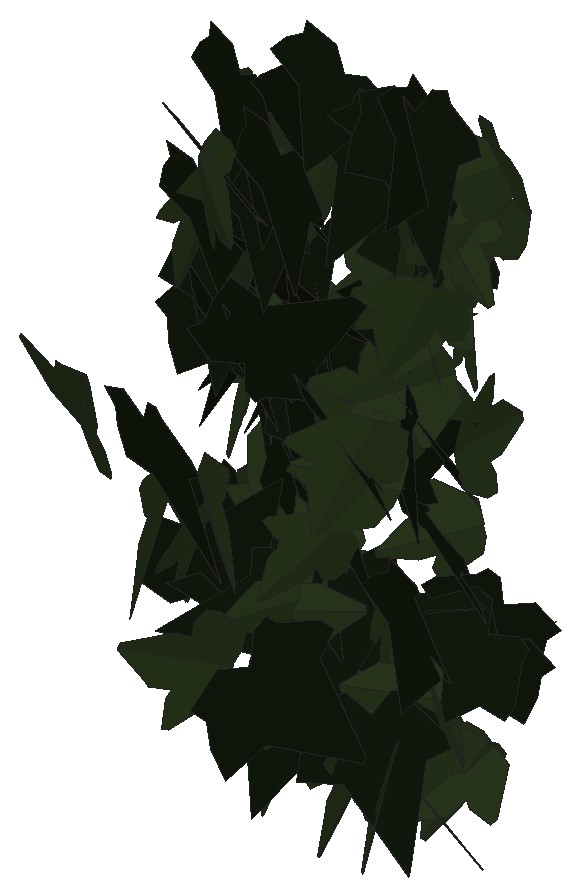
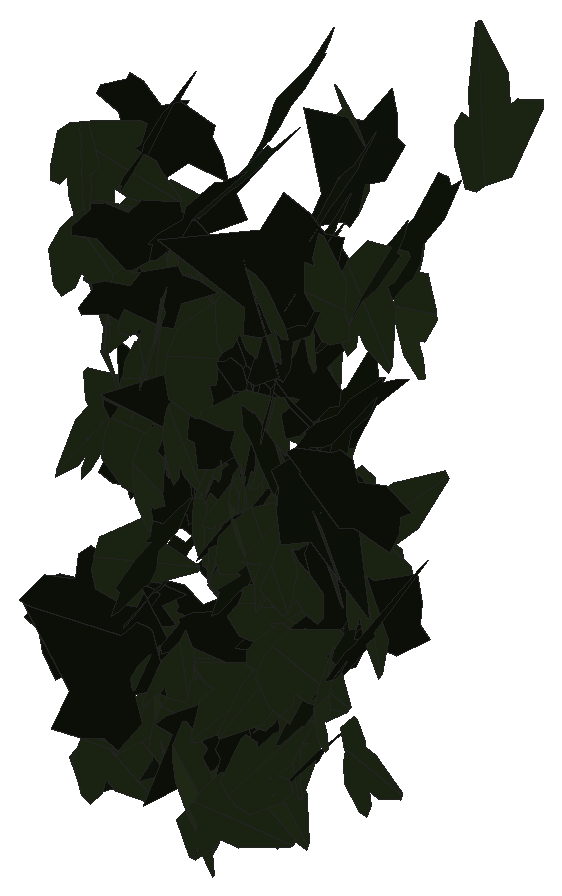
# SketchUp Ruby script. Lengths in inches.
U = 1.inch
M = Sketchup.active_model
def pt(a) = Geom::Point3d.new(a.map { |v| v * U })
def face(e, loops, mat)
  f = e.add_face(loops[0].map { |a| pt(a) })
  loops[1..].each { |l| e.add_face(l.map { |a| pt(a) }).erase! }
  f.material = f.back_material = mat if mat
  f
end
# faces: each face lists its corners as indices into pts; further lists are holes
def faces(e, pts, list, mat = nil) = list.each { |f| face(e, (f[0].is_a?(Array) ? f : [f]).map { |l| l.map { |i| pts[i] } }, mat) }
# xy, xz, yz: faces in a plane at the given z, y or x. An outline is a flat list of corners, or four numbers for a rectangle; further outlines are holes
def ring(l) = l.size == 4 ? [[l[0], l[1]], [l[2], l[1]], [l[2], l[3]], [l[0], l[3]]] : l.each_slice(2).to_a
def flat(e, list, mat, &to3) = list.each { |f| face(e, (f[0].is_a?(Array) ? f : [f]).map { |l| ring(l).map { |u, v| to3.(u, v) } }, mat) }
def xy(e, z, list, mat = nil) = flat(e, list, mat) { |x, y| [x, y, z] }
def xz(e, y, list, mat = nil) = flat(e, list, mat) { |x, z| [x, y, z] }
def yz(e, x, list, mat = nil) = flat(e, list, mat) { |y, z| [x, y, z] }
def lines(e, pts, list) = list.each { |a, b| e.add_line(pt(pts[a]), pt(pts[b])) }
# prism: a flat outline (further loops are holes) pulled along v
def prism(e, loops, v, mat = nil)
  f = face(e, loops, mat); d = Geom::Vector3d.new(v.map { |x| x * U })
  f.pushpull(f.normal.samedirection?(d) ? d.length : -d.length)
end
def box(e, o, s, mat = nil) = prism(e, [[o, [o[0] + s[0], o[1], o[2]], [o[0] + s[0], o[1] + s[1], o[2]], [o[0], o[1] + s[1], o[2]]]], [0, 0, s[2]], mat)
def at(x, y, z, deg = 0) = Geom::Transformation.translation(pt([x, y, z])) * Geom::Transformation.rotation(ORIGIN, Z_AXIS, deg.degrees)
def axes(o, x, y, z) = Geom::Transformation.new([*x, 0, *y, 0, *z, 0, *pt(o).to_a, 1])
def part(name) = M.definitions.add(name)
# library, detail: a bought-in or finely detailed component or shape, given as its bounding box
def library(name, o, s) = part(name).tap { |d| box(d.entities, o, s) }
def detail(e, o, s) = box(e.add_group.entities, o, s)
def put(e, d, t, mat = nil) = e.add_instance(d, t).tap { |i| i.material = mat if mat }
def group(e, t, mat = nil) = e.add_group.tap { |g| g.transformation = t; g.material = mat if mat }.entities
root = M.entities
M.materials.add("efeu1").color = [18, 25, 13]
M.materials.add("efeu2").color = [43, 57, 29]
c1 = part("ivyleaf_10")
p = [[0,0.5,-0.03],[-0.0625,2.02,-0.43],[-0.19,2.01,-0.46],[-0.54,1.05,-0.29],[-0.52,0.625,-0.18],[-0.83,0.76,-0.28],
  [-1.16,0.64,-0.33],[-1.15,0.33,-0.24],[-0.77,-0.39,0.02],[-0.3,-0.51,0.16],[0.04,-0.48,0.23],[-0.02,2.01,-0.4375],
  [-0.06,2.01,-0.43],[0.04,-0.49,0.23],[0.67,-0.49,0.14],[1.38,0.36,-0.2],[1.375,0.51,-0.24],[0.81,0.65,-0.19],
  [0.62,0.59,-0.15],[0.6,1.09,-0.28],[0.5,1.23,-0.31]]
faces(c1.entities,p,[[0,1,2,3,4,5,6,7,8,9,10],[11,12,0,13,14,15,16,17,18,19,20]],"efeu2")
c2 = part("ivyleaf_9")
p = [[1.54,2.16,1.25],[1.36,2.04,1.19],[-0.21,0.99,0.68],[-0.71,1.11,0.82],[-0.85,0.86,0.67],[-0.8,0.17,0.21],
  [-0.9,-0.01,0.1],[-0.67,-0.16,-0.02],[-0.08,-0.08,-0.05],[-0.03,-0.6,-0.4],[0.65,-0.88,-0.66],[0.83,-0.6,-0.49],
  [1.29,-0.42,-0.43],[1.8125,-0.07,-0.26],[1.21,0.44,0.15]]
faces(c2.entities,p,[[0,1,2,3,4,5,6,7,8,9,10,11,12,13,14]],"efeu1")
put(root,c1,axes([521.53,128.375,181.19],[-0.85624,0.15048,0.62072],[0.56209,-0.31547,0.85184],[0.30331,1.00942,0.17368]))
put(root,c1,axes([521.82,130.08,178.96],[0.25692,-0.3956,0.84112],[0.51271,-0.66758,-0.47059],[0.77531,0.57256,0.03248]))
put(root,c2,axes([521.51,130.16,180.27],[0.564,-0.75753,0.18315],[0.11068,-0.14594,-0.94443],[0.77146,0.57475,0.0016]))
put(root,c1,axes([521.68,131.56,175.45],[-0.18984,-0.2558,-0.80001],[-0.49065,-0.63191,0.31848],[-0.68169,0.52606,-0.00644]))
put(root,c2,axes([522.62,131.46,175.6875],[0.12859,-0.32835,-0.91099],[-0.21634,0.88602,-0.34989],[0.94388,0.24781,0.04391]))
put(root,c1,axes([521.26,132.04,178.09],[-0.47981,0.69752,0.08512],[-0.04953,0.06925,-0.84661],[-0.70095,-0.48236,0.00156]))
put(root,c1,axes([520.76,132.68,183.39],[-0.20173,0.08556,-0.81779],[0.49347,-0.66094,-0.19087],[-0.65771,-0.52214,0.10761]))
put(root,c1,axes([523.77,132.73,179.65],[-0.39116,-0.67084,0.38941],[-0.11622,-0.38051,-0.77226],[0.76692,-0.39982,0.08158]))
put(root,c2,axes([521.96,132.93,183.94],[0.23926,-0.74582,0.36603],[0.08109,-0.35812,-0.78272],[0.82683,0.25094,-0.02915]))
put(root,c2,axes([522.88,133.11,179.41],[0.29561,-0.55547,0.55692],[0.36081,-0.43291,-0.6233],[0.69894,0.45841,0.08621]))
put(root,c2,axes([520.23,133.24,183.27],[0.22099,-0.49408,0.66016],[0.45648,-0.49587,-0.52393],[0.6867,0.48863,0.13583]))
put(root,c1,axes([523.62,133.49,173.44],[0.53015,-0.61555,0.24235],[0.15312,-0.18795,-0.81236],[0.64357,0.55179,-0.00635]))
put(root,c2,axes([521.26,133.03,180.08],[-0.05232,-0.01524,0.84946],[0.84681,-0.06992,0.0509],[0.06887,0.8482,0.01946]))
put(root,c2,axes([523.47,133.32,174.27],[-0.36679,-0.49197,-0.58723],[0.35546,0.46744,-0.61364],[0.67862,-0.51076,0.00403]))
put(root,c1,axes([522.92,133.78,173.35],[0.22016,-0.65504,0.51825],[0.17005,-0.48957,-0.69103],[0.81776,0.27815,0.00417]))
put(root,c1,axes([522.21,133.6875,176.93],[-0.25975,-0.43298,0.49778],[-0.24936,-0.43086,-0.50489],[0.6108,-0.36003,0.00557]))
put(root,c1,axes([523.02,133.96,178.05],[0.04142,0.41072,0.69902],[-0.12808,-0.68783,0.41173],[0.80057,-0.1313,0.0297]))
put(root,c1,axes([521.35,134.22,175.35],[0.00535,0.07548,0.79166],[-0.02054,-0.7914,0.07559],[0.79498,-0.02096,-0.00338]))
put(root,c2,axes([521.42,134.17,175.21],[-0.12864,-0.31702,-0.71842],[-0.31596,-0.64557,0.34145],[-0.71889,0.34046,-0.02151]))
put(root,c1,axes([519.73,133.77,176.43],[0.13839,-0.83853,-0.06256],[-0.01138,0.06153,-0.84988],[0.84079,0.13885,-0.0012]))
put(root,c2,axes([519.41,134.3,181.83],[0.19789,-0.72797,0.42536],[0.17769,-0.3911,-0.752],[0.8242,0.2591,0.06]))
put(root,c2,axes([519.8,133.7,175.1875],[-0.37067,-0.1078,0.73364],[0.73908,-0.12015,0.35576],[0.06007,0.81313,0.14983]))
put(root,c1,axes([523.99,133.98,181.66],[-0.52596,-0.47765,0.32754],[-0.24717,-0.21501,-0.71046],[0.52378,-0.58111,-0.00636]))
put(root,c1,axes([521.04,133.76,173.81],[0.07599,-0.79622,-0.29415],[-0.03191,0.29244,-0.79983],[0.84822,0.08233,-0.00374]))
put(root,c1,axes([519.47,134.27,182.06],[0.10925,-0.81636,0.27169],[0.07847,-0.26328,-0.82263],[0.8568,0.1282,0.0407]))
put(root,c1,axes([520.4,134.18,181.11],[0.20781,-0.69335,0.09716],[0.03159,-0.09196,-0.72381],[0.69941,0.21017,0.00383]))
put(root,c2,axes([520.39,134.51,182.125],[0.08087,-0.70528,0.31233],[0.07837,-0.3049,-0.7088],[0.76735,0.10547,0.03947]))
put(root,c1,axes([520.95,134.02,175.13],[0.15316,-0.01523,-0.79976],[0.79856,-0.04419,0.15377],[-0.04627,-0.81309,0.00662]))
put(root,c1,axes([522.4,134.49,178.82],[-0.13144,0.57468,0.54752],[0.08748,-0.5411,0.58895],[0.78891,0.15575,0.02591]))
put(root,c1,axes([523.69,134.3,174.36],[-0.09119,0.13167,0.69466],[-0.66242,-0.26077,-0.03753],[0.24717,-0.65028,0.1557]))
put(root,c2,axes([523.26,134.86,175.35],[-0.05277,-0.63435,0.54605],[0.13533,-0.5464,-0.62168],[0.82599,0.049,0.13674]))
put(root,c2,axes([520.5,134.83,172.75],[-0.09164,-0.66778,0.37274],[0.0439,-0.37939,-0.66888],[0.7635,-0.05834,0.0832]))
put(root,c2,axes([521.42,134.74,173.29],[0.21327,-0.59262,0.45455],[0.21942,-0.40214,-0.62724],[0.71391,0.30063,0.057]))
put(root,c2,axes([519.59,134.86,183.74],[0.10259,-0.63407,0.45046],[0.06087,-0.44642,-0.64225],[0.7754,0.11893,-0.00918]))
put(root,c2,axes([519.35,134.69,179.61],[0.41128,-0.63319,0.40762],[0.23052,-0.33629,-0.75498],[0.7169,0.47139,0.00892]))
put(root,c1,axes([522.7,134.83,178.26],[0.05596,-0.34727,0.61371],[0.20579,-0.5808,-0.34741],[0.67445,0.20603,0.05508]))
put(root,c2,axes([520.7,134.9,174.8],[-0.06086,-0.62189,-0.43502],[-0.0524,-0.43193,0.62481],[-0.75713,0.07989,-0.00827]))
put(root,c1,axes([519.6,134.26,173.23],[0.04765,0.02788,0.68359],[-0.68078,0.06996,0.0446],[-0.06792,-0.68167,0.03253]))
put(root,c1,axes([520.6875,134.84,172.67],[0.18984,-0.66091,0.34813],[0.14198,-0.32073,-0.68631],[0.73338,0.23317,0.04275]))
put(root,c1,axes([522.44,135.08,173.35],[-0.25909,-0.3786,0.71299],[-0.13826,-0.71693,-0.43094],[0.79535,-0.24796,0.15735]))
put(root,c2,axes([523.13,135.23,183.72],[-0.03538,-0.57911,0.57544],[-0.05395,-0.57307,-0.58004],[0.81462,-0.06311,-0.01342]))
put(root,c2,axes([522.87,134.52,172.9],[0.71397,-0.31497,0.00674],[0.00939,0.0046,-0.78032],[0.3149,0.71399,0.008]))
put(root,c1,axes([523.03,134.8125,173.31],[0.26524,-0.63065,0.18301],[0.09335,-0.15916,-0.68375],[0.65,0.28021,0.02352]))
put(root,c1,axes([523.98,134.4,174.46],[-0.35506,0.58791,0.17196],[-0.08336,0.15054,-0.68678],[-0.60685,-0.36466,-0.00628]))
put(root,c2,axes([523.12,134.81,184.26],[-0.49904,-0.31405,-0.64784],[0.56056,0.32513,-0.58942],[0.45176,-0.75035,0.01574]))
put(root,c2,axes([524.24,135.11,175.24],[-0.79644,-0.34036,0.05383],[-0.04794,-0.02479,-0.86611],[0.34124,-0.79787,0.00395]))
put(root,c2,axes([519.77,135.26,182.63],[0.1517,-0.66109,0.46611],[0.08104,-0.45943,-0.67798],[0.80482,0.17087,-0.01959]))
put(root,c2,axes([521.63,135.12,175.625],[-0.26911,-0.80421,-0.07446],[0.03559,0.0666,-0.84795],[0.80686,-0.27116,0.01257]))
put(root,c1,axes([523.21,135.13,179.45],[0.12505,0.11534,-0.73489],[-0.57248,-0.46092,-0.16976],[-0.47501,0.58587,0.01113]))
put(root,c2,axes([521.02,135.02,176.93],[0.46228,-0.63508,0.26605],[0.15765,-0.21431,-0.78551],[0.67026,0.48843,0.00126]))
put(root,c2,axes([519.93,134.68,180.57],[0.68497,-0.22833,0.42596],[0.41191,-0.11064,-0.7217],[0.25279,0.79899,0.02179]))
put(root,c2,axes([519.31,135.14,175.24],[0.06929,-0.84181,0.0159],[0.0358,0.01889,0.84384],[-0.8412,-0.06854,0.03722]))
put(root,c2,axes([519.52,135.1875,175],[0.29982,-0.68673,0.3923],[0.19137,-0.34408,-0.74858],[0.76738,0.35412,0.03341]))
put(root,c2,axes([519.13,135.21,180.1875],[-0.07882,-0.76088,0.06984],[0.00722,-0.07095,-0.76481],[0.76404,-0.07782,0.01443]))
put(root,c2,axes([521.05,134.41,177.35],[-0.02375,0.05329,0.85173],[-0.4074,0.74799,-0.05816],[-0.74987,-0.40807,0.00462]))
put(root,c2,axes([521.74,135.3,178.01],[-0.13584,-0.26803,0.76169],[0.34942,-0.71584,-0.18958],[0.72795,0.29359,0.23314]))
put(root,c2,axes([522.52,135.09,178.88],[-0.1911,-0.02871,-0.79209],[0.79199,-0.03908,-0.18966],[-0.03128,-0.81388,0.03705]))
put(root,c2,axes([520.92,135.21,179.64],[0.07488,-0.04378,-0.84611],[0.82932,-0.16998,0.08219],[-0.17332,-0.83223,0.02772]))
put(root,c2,axes([522.91,135.23,178.45],[0.62661,-0.09736,-0.53106],[0.51982,-0.11112,0.63371],[-0.14594,-0.81383,-0.023]))
put(root,c2,axes([520.33,135.375,180.45],[0.22772,-0.13195,-0.80412],[0.73488,-0.32752,0.26185],[-0.35211,-0.76889,0.02646]))
put(root,c1,axes([520.42,134.38,181.75],[0.24535,-0.40291,-0.73346],[-0.04858,0.75618,-0.43165],[0.83542,0.1623,0.19031]))
put(root,c1,axes([523.3,135.27,180.86],[0.17693,0.46418,-0.50116],[-0.19939,-0.46006,-0.49651],[-0.65336,0.2661,0.0158]))
put(root,c2,axes([520.6,134.75,179.52],[-0.54444,0.47702,0.31955],[0.24274,-0.20784,0.72385],[0.52033,0.59609,-0.00333]))
put(root,c2,axes([521,135.64,183.91],[-0.16398,-0.64872,0.4484],[0.1046,-0.47184,-0.64438],[0.78164,-0.07295,0.1803]))
put(root,c1,axes([521.34,135.05,175.8125],[0.25429,0.19286,0.61867],[-0.6057,-0.16551,0.30056],[0.23035,-0.64809,0.10735]))
put(root,c2,axes([521.97,135.61,183],[-0.22643,-0.70313,0.32913],[-0.09452,-0.31533,-0.73866],[0.77057,-0.24529,0.00611]))
put(root,c1,axes([522.89,135.04,180.95],[-0.32006,-0.61883,-0.10988],[0.0748,0.08493,-0.69617],[0.62404,-0.32757,0.02709]))
put(root,c1,axes([523.0625,135.62,178.73],[-0.15991,-0.41095,0.66463],[-0.08411,-0.66541,-0.43167],[0.77687,-0.15663,0.09007]))
put(root,c1,axes([523.73,135.49,172.74],[0.28446,0.31832,-0.64202],[-0.40644,-0.49723,-0.42662],[-0.59019,0.49585,-0.01565]))
put(root,c1,axes([523.97,135.37,183.36],[-0.29626,-0.13598,0.66689],[-0.51236,-0.43421,-0.31615],[0.44802,-0.58649,0.07944]))
put(root,c2,axes([521.19,135.04,179.76],[-0.18781,-0.20371,-0.74298],[0.55065,0.49935,-0.2761],[0.53881,-0.58133,0.02319]))
put(root,c1,axes([523.04,134.74,173.8],[-0.09605,-0.46352,-0.58755],[0.19105,0.55755,-0.47108],[0.72357,-0.20874,0.04639]))
put(root,c1,axes([521.76,135.77,180.54],[-0.04695,-0.26694,0.78899],[0.04413,-0.78992,-0.26463],[0.83175,0.02684,0.05858]))
put(root,c1,axes([521.5625,135.66,177.96],[0.03462,-0.40899,0.67144],[0.4572,-0.53629,-0.35024],[0.63959,0.40549,0.21402]))
put(root,c2,axes([524.2,135.42,175],[0.10849,0.17324,-0.78605],[-0.37655,-0.69008,-0.20406],[-0.7114,0.39169,-0.01186]))
put(root,c1,axes([521.05,135.02,178.64],[-0.60688,0.13325,0.44916],[-0.43678,0.10498,-0.6213],[-0.16948,-0.74768,-0.00718]))
put(root,c1,axes([523.67,135.59,172.6875],[-0.19456,-0.54533,0.44438],[-0.04012,-0.45172,-0.57189],[0.70232,-0.17687,0.09044]))
put(root,c1,axes([521.95,135.09,178.76],[-0.59964,0.36286,0.0569],[-0.05373,0.02109,-0.70081],[-0.36334,-0.60196,0.00974]))
put(root,c2,axes([522.04,135.25,177.68],[-0.0044,0.01,0.7808],[0.69355,-0.35873,0.0085],[0.35881,0.69353,-0.00686]))
put(root,c1,axes([522.81,134.87,181.83],[0.33113,-0.44636,-0.5607],[-0.06927,0.59483,-0.51444],[0.71331,0.26497,0.21032]))
put(root,c1,axes([521.46,135.18,172.46],[-0.50566,0.46782,-0.06119],[0.04016,-0.04669,-0.68883],[-0.47009,-0.5072,0.00697]))
put(root,c1,axes([519.92,135.39,177.16],[0.56142,-0.05936,0.54914],[0.5484,-0.0334,-0.56427],[0.06582,0.78462,0.01753]))
put(root,c1,axes([520.51,135.22,179.75],[0.57948,0.51038,0.1776],[0.12641,0.12515,-0.77213],[-0.52541,0.59302,0.0101]))
put(root,c2,axes([520.62,135.46,179.69],[-0.63044,0.38707,-0.37531],[0.31933,-0.19719,-0.73978],[-0.43441,-0.7067,0.00086]))
put(root,c1,axes([519.33,135.49,178.29],[0.54759,-0.58363,0.08434],[0.05288,-0.06604,-0.80027],[0.58731,0.5501,-0.00659]))
put(root,c2,axes([520.65,135.61,178.08],[0.1058,-0.77584,-0.03838],[0.00074,0.03884,-0.783],[0.77679,0.10564,0.00598]))
put(root,c2,axes([519.77,135.67,181.58],[0.28081,-0.43337,0.59863],[0.37955,-0.46491,-0.51461],[0.63412,0.47019,0.04292]))
put(root,c2,axes([521.2,134.95,173.66],[0.23786,-0.24765,-0.71149],[-0.49991,0.50629,-0.34335],[0.5636,0.55359,-0.00427]))
put(root,c2,axes([524.14,135.64,175.51],[0.07964,0.15391,-0.78659],[-0.30516,-0.7251,-0.17277],[-0.74113,0.3151,-0.01338]))
put(root,c1,axes([523.27,135.39,182.17],[-0.57183,-0.15728,-0.38861],[0.4161,-0.13262,-0.5586],[0.05122,-0.67855,0.19926]))
put(root,c2,axes([521.32,135.21,173.82],[0.05042,-0.48785,-0.65914],[0.15184,0.65451,-0.47282],[0.80586,-0.09281,0.13033]))
put(root,c1,axes([522.17,135.55,174.91],[-0.01682,0.64786,-0.29071],[-0.0117,-0.291,-0.64784],[-0.70999,-0.01055,0.01756]))
put(root,c1,axes([519.74,135.76,175.67],[-0.27186,-0.36538,0.50238],[-0.21471,-0.45932,-0.45025],[0.58292,-0.33959,0.06846]))
put(root,c2,axes([519.5,135.36,178.95],[-0.3204,0.70546,-0.28972],[0.12334,-0.26218,-0.7748],[-0.7526,-0.34331,-0.00364]))
put(root,c1,axes([522.95,135.29,180.26],[-0.43648,0.55166,0.04397],[-0.02795,0.03394,-0.70345],[-0.5527,-0.43738,0.00086]))
put(root,c1,axes([520.75,135.8,178.125],[0.30861,-0.40224,0.49839],[0.32754,-0.37629,-0.50651],[0.55037,0.44949,0.02198]))
put(root,c1,axes([520.67,135.68,182.06],[-0.17379,-0.67208,0.2436],[0.01197,-0.2534,-0.69056],[0.71476,-0.15917,0.0708]))
put(root,c2,axes([521.24,135.03,179.53],[0.33687,0.10623,0.71943],[0.67758,0.24209,-0.35302],[-0.26411,0.7566,0.01195]))
put(root,c1,axes([523.58,135.44,182.01],[-0.47297,-0.5253,-0.05863],[0.04094,0.04204,-0.70684],[0.52697,-0.47473,0.00228]))
put(root,c1,axes([521.32,135.4,178.12],[-0.62388,0.31113,-0.01822],[0.01713,-0.00648,-0.69715],[-0.31119,-0.62411,-0.00184]))
put(root,c2,axes([518.58,135.49,179.24],[-0.09137,-0.30954,-0.73597],[0.55506,0.50785,-0.28251],[0.57391,-0.54045,0.15606]))
put(root,c1,axes([521.96,135.18,171.8],[-0.21816,0.25712,-0.62747],[-0.38004,0.49953,0.33683],[0.5616,0.43792,-0.01581]))
put(root,c1,axes([518.92,135.63,182.53],[0.06903,-0.02856,0.7653],[0.76583,0.00278,-0.06898],[-0.0002,0.7684,0.0287]))
put(root,c1,axes([520.41,135.96,173.28],[0.03048,0.38157,0.59939],[-0.00296,-0.59986,0.38202],[0.71053,-0.01887,-0.02413]))
put(root,c1,axes([523.125,135.97,176.42],[-0.12407,-0.02979,0.65734],[-0.30981,-0.58749,-0.0851],[0.58052,-0.3199,0.09508]))
put(root,c2,axes([522.8,135.94,181.58],[-0.42724,-0.61226,-0.13834],[0.07645,0.11534,-0.74658],[0.62302,-0.43401,-0.00325]))
put(root,c2,axes([522.38,135.88,176.83],[0.47351,-0.63218,0.24455],[0.16592,-0.18113,-0.78952],[0.65721,0.50121,0.02313]))
put(root,c1,axes([523.75,135.99,182.22],[-0.31593,-0.56594,0.40793],[-0.04566,-0.43008,-0.63202],[0.69614,-0.28505,0.14368]))
put(root,c2,axes([522.86,135.94,182.89],[-0.4414,-0.55364,-0.28117],[0.16997,0.22407,-0.70803],[0.59723,-0.47295,-0.00631]))
put(root,c1,axes([522.4,136.16,178.41],[0.20505,-0.45579,0.53559],[0.30825,-0.4432,-0.49518],[0.63213,0.36397,0.06773]))
put(root,c1,axes([523.14,136.08,180.29],[0.25122,-0.17501,0.64405],[0.55307,-0.33057,-0.30556],[0.37355,0.60715,0.01928]))
put(root,c1,axes([521.05,135.48,178.15],[-0.21027,0.65568,0.24164],[-0.08356,0.22694,-0.68851],[-0.69378,-0.22606,0.00969]))
put(root,c1,axes([518.74,136.17,175.35],[0.07902,-0.18303,0.63821],[0.44891,-0.45882,-0.18716],[0.48918,0.45061,0.06866]))
put(root,c1,axes([519.98,135.54,177.8125],[-0.07313,0.64881,0.20442],[-0.01464,0.20405,-0.65287],[-0.68009,-0.07416,-0.00793]))
put(root,c2,axes([519.6875,135.53,182.58],[0.29514,0.01489,0.76499],[0.76513,-0.00178,-0.29516],[-0.0037,0.81995,-0.01453]))
put(root,c1,axes([520.28,135.88,182.4],[0.63626,-0.47483,-0.06576],[-0.04701,0.04695,-0.79385],[0.47706,0.63792,0.00948]))
put(root,c1,axes([524.22,135.63,183.57],[-0.57123,0.24738,0.35267],[-0.3429,0.09344,-0.62094],[-0.26076,-0.6648,0.04395]))
put(root,c1,axes([520.3,135.89,177.94],[-0.58533,-0.2549,0.30708],[-0.26418,-0.16111,-0.63729],[0.29914,-0.64106,0.03806]))
put(root,c1,axes([523.96,135.23,178.5],[-0.03191,0.07864,0.80259],[-0.31926,0.73636,-0.08484],[-0.74055,-0.32084,0.002]))
put(root,c1,axes([521.74,136.1,179.49],[0.17612,-0.66475,0.24323],[0.10443,-0.2235,-0.68645],[0.70011,0.20056,0.04121]))
put(root,c1,axes([521.52,136.17,173.34],[0.33923,-0.65328,0.32352],[0.12777,-0.29803,-0.73578],[0.71771,0.36183,-0.02193]))
put(root,c1,axes([520.21,135.32,175.31],[-0.09337,-0.37706,-0.74177],[0.20384,0.71331,-0.38825],[0.80674,-0.22388,0.01225]))
put(root,c2,axes([523.1,135.64,173.87],[0.48716,0.54428,-0.20873],[0.0859,0.20202,0.72728],[0.57657,-0.48998,0.068]))
put(root,c1,axes([520.59,135.65,174.8],[0.34931,0.33498,0.47907],[0.32086,0.35663,-0.48332],[-0.48864,0.47364,0.0251]))
put(root,c1,axes([520.88,136.25,172.79],[0.35768,0.26909,-0.60779],[-0.48861,-0.3615,-0.44759],[-0.45065,0.60553,0.00289]))
